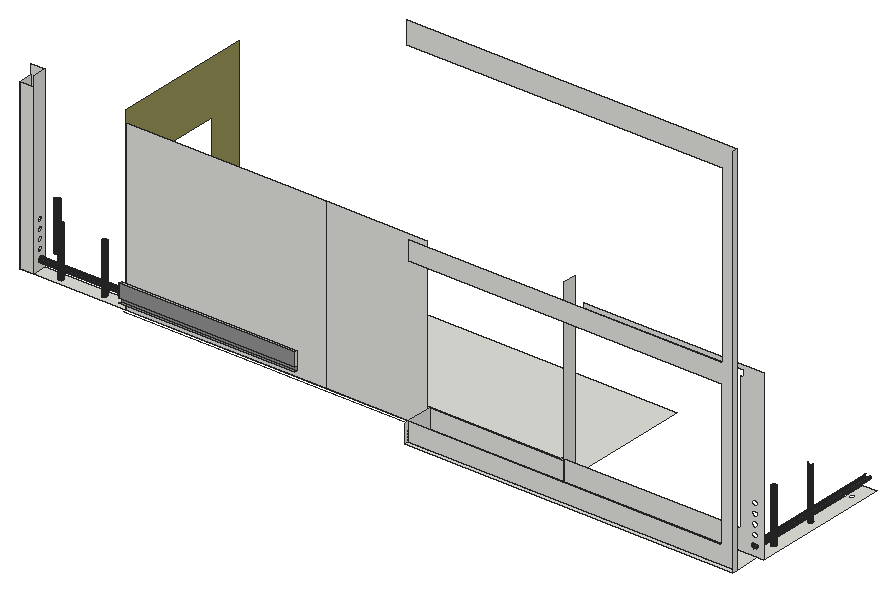
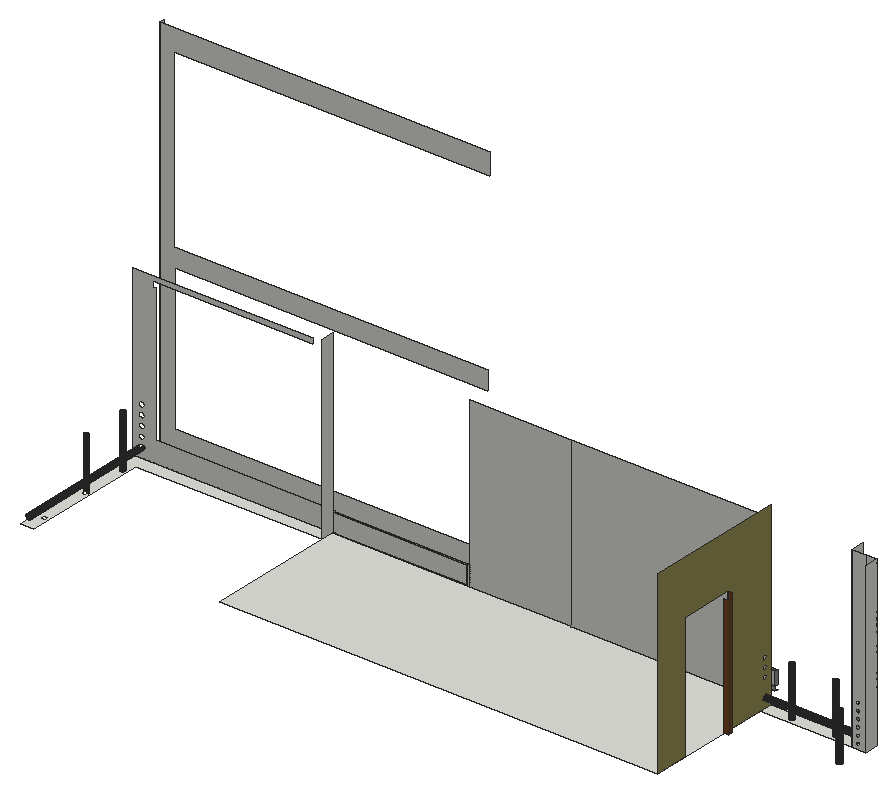
# SketchUp Ruby script. Lengths in inches.
U = 1.inch
M = Sketchup.active_model
def pt(a) = Geom::Point3d.new(a.map { |v| v * U })
def face(e, loops, mat)
  f = e.add_face(loops[0].map { |a| pt(a) })
  loops[1..].each { |l| e.add_face(l.map { |a| pt(a) }).erase! }
  f.material = f.back_material = mat if mat
  f
end
# faces: each face lists its corners as indices into pts; further lists are holes
def faces(e, pts, list, mat = nil) = list.each { |f| face(e, (f[0].is_a?(Array) ? f : [f]).map { |l| l.map { |i| pts[i] } }, mat) }
# xy, xz, yz: faces in a plane at the given z, y or x. An outline is a flat list of corners, or four numbers for a rectangle; further outlines are holes
def ring(l) = l.size == 4 ? [[l[0], l[1]], [l[2], l[1]], [l[2], l[3]], [l[0], l[3]]] : l.each_slice(2).to_a
def flat(e, list, mat, &to3) = list.each { |f| face(e, (f[0].is_a?(Array) ? f : [f]).map { |l| ring(l).map { |u, v| to3.(u, v) } }, mat) }
def xy(e, z, list, mat = nil) = flat(e, list, mat) { |x, y| [x, y, z] }
def xz(e, y, list, mat = nil) = flat(e, list, mat) { |x, z| [x, y, z] }
def yz(e, x, list, mat = nil) = flat(e, list, mat) { |y, z| [x, y, z] }
def lines(e, pts, list) = list.each { |a, b| e.add_line(pt(pts[a]), pt(pts[b])) }
# prism: a flat outline (further loops are holes) pulled along v
def prism(e, loops, v, mat = nil)
  f = face(e, loops, mat); d = Geom::Vector3d.new(v.map { |x| x * U })
  f.pushpull(f.normal.samedirection?(d) ? d.length : -d.length)
end
def box(e, o, s, mat = nil) = prism(e, [[o, [o[0] + s[0], o[1], o[2]], [o[0] + s[0], o[1] + s[1], o[2]], [o[0], o[1] + s[1], o[2]]]], [0, 0, s[2]], mat)
def at(x, y, z, deg = 0) = Geom::Transformation.translation(pt([x, y, z])) * Geom::Transformation.rotation(ORIGIN, Z_AXIS, deg.degrees)
def axes(o, x, y, z) = Geom::Transformation.new([*x, 0, *y, 0, *z, 0, *pt(o).to_a, 1])
def part(name) = M.definitions.add(name)
# library, detail: a bought-in or finely detailed component or shape, given as its bounding box
def library(name, o, s) = part(name).tap { |d| box(d.entities, o, s) }
def detail(e, o, s) = box(e.add_group.entities, o, s)
def put(e, d, t, mat = nil) = e.add_instance(d, t).tap { |i| i.material = mat if mat }
def group(e, t, mat = nil) = e.add_group.tap { |g| g.transformation = t; g.material = mat if mat }.entities
root = M.entities
M.materials.add("[0057_DarkKhaki]").color = [150, 145, 85]
M.materials.add("[0137_Black]").color = [71, 71, 71]
M.materials.add("[Color M05]").color = [145, 145, 145]
M.materials.add("[Wood Veneer 01]").color = [120, 70, 37]
xy(root,123,[[11.875,22.0625,20.875,31.0625],[[20.875,22.0625,82.85,31.0625],[35.53,25.16,35.13,25.24,34.76,25.43,34.46,25.7,34.23,26.04,34.1,26.42,34.08,26.83,34.16,27.23,34.34,27.59,34.61,27.9,34.95,28.125,35.34,28.25,35.75,28.28,36.15,28.2,36.51,28.02,36.82,27.75,37.04,27.41,37.17,27.02,37.2,26.61,37.11,26.21,36.93,25.85,36.66,25.54,36.32,25.32,35.9375,25.1875],[64.53,25.16,64.13,25.24,63.76,25.43,63.46,25.7,63.23,26.04,63.1,26.42,63.08,26.83,63.16,27.23,63.34,27.59,63.61,27.9,63.95,28.125,64.34,28.25,64.75,28.28,65.15,28.2,65.51,28.02,65.82,27.75,66.04,27.41,66.17,27.02,66.2,26.61,66.11,26.21,65.93,25.85,65.66,25.54,65.32,25.32,64.9375,25.1875]],[82.85,22.0625,376.99,116.75],[[376.99,22.0625,510.6875,22.0625,510.6875,116.75,501.6875,116.75,501.6875,31.0625,376.99,31.0625],[504.72,36.55,504.27,36.6,503.85,36.78,503.49,37.06,503.21,37.42,503.03,37.84,502.97,38.3,503.03,38.75,503.21,39.17,503.49,39.53,503.85,39.8125,504.27,39.99,504.72,40.05,505.18,39.99,505.6,39.8125,505.96,39.53,506.24,39.17,506.41,38.75,506.47,38.3,506.41,37.84,506.24,37.42,505.96,37.06,505.6,36.78,505.18,36.6],[504.72,67.92,504.27,67.98,503.85,68.15,503.49,68.43,503.21,68.8,503.03,69.22,502.97,69.67,503.03,70.125,503.21,70.55,503.49,70.91,503.85,71.1875,504.27,71.36,504.72,71.42,505.18,71.36,505.6,71.1875,505.96,70.91,506.24,70.55,506.41,70.125,506.47,69.67,506.41,69.22,506.24,68.8,505.96,68.43,505.6,68.15,505.18,67.98],[504.72,102.17,504.27,102.23,503.85,102.4,503.49,102.68,503.21,103.05,503.03,103.47,502.97,103.92,503.03,104.375,503.21,104.8,503.49,105.16,503.85,105.4375,504.27,105.61,504.72,105.67,505.18,105.61,505.6,105.4375,505.96,105.16,506.24,104.8,506.41,104.375,506.47,103.92,506.41,103.47,506.24,103.05,505.96,102.68,505.6,102.4,505.18,102.23]],[79.85,58.11,82.85,61.11]])
xy(root,123.19,[[286.64,1.0625,507.04,4.0625],[286.64,4.0625,507.04,22.0625]])
xy(root,129.65,[[82.85,16.375,200.79,18.1875]],"[Color M05]")
xy(root,132.55,[[82.85,16.375,200.79,18.1875]])
xz(root,4.0625,[[286.64,123.19,507.04,123.19,507.04,376.42,285.64,376.42,285.64,361.64,497.49,361.64,497.49,244.84,286.99,244.84,286.99,232.22,497.29,232.22,497.29,135.48,286.64,135.48]])
xz(root,16.375,[[82.85,132.55,200.79,141.65]],"[Color M05]")
xz(root,18.1875,[[82.85,132.55,200.79,141.65]])
xz(root,18.1875,[[82.85,129.65,200.79,132.55]],"[Color M05]")
xz(root,22.0625,[[11.875,123,20.875,235.42],[82.85,123,216.73,235.42],[216.73,123,216.79,235.42],[216.79,123,284.41,235.42],[284.41,123,376.99,123,376.99,123.19,286.64,123.19,286.64,135.48,376.99,135.48,376.99,137.03,375.29,137.03,375.29,135.98,284.41,135.98],
  [[376.99,123,376.99,137.03,495.71,137.03,495.71,228.47,497.29,228.47,497.29,232.22,390.0625,232.22,390.0625,235.42,510.6875,235.42,510.6875,123],[504.95,127.5625,505.43,127.625,505.88,127.8125,506.27,128.11,506.57,128.5,506.76,128.95,506.82,129.4375,506.76,129.92,506.57,130.375,506.27,130.76,505.88,131.0625,505.43,131.25,504.95,131.3125,504.46,131.25,504.01,131.0625,503.62,130.76,503.32,130.375,503.14,129.92,503.07,129.4375,503.14,128.95,503.32,128.5,503.62,128.11,504.01,127.8125,504.46,127.625],[504.95,134,505.43,134.0625,505.88,134.25,506.27,134.55,506.57,134.9375,506.76,135.39,506.82,135.875,506.76,136.36,506.57,136.8125,506.27,137.2,505.88,137.5,505.43,137.69,504.95,137.75,504.46,137.69,504.01,137.5,503.62,137.2,503.32,136.8125,503.14,136.36,503.07,135.875,503.14,135.39,503.32,134.9375,503.62,134.55,504.01,134.25,504.46,134.0625],[504.95,140.4375,505.43,140.5,505.88,140.6875,506.27,140.99,506.57,141.375,506.76,141.83,506.82,142.3125,506.76,142.8,506.57,143.25,506.27,143.64,505.88,143.9375,505.43,144.12,504.95,144.1875,504.46,144.12,504.01,143.9375,503.62,143.64,503.32,143.25,503.14,142.8,503.07,142.3125,503.14,141.83,503.32,141.375,503.62,140.99,504.01,140.6875,504.46,140.5],[504.95,146.875,505.43,146.9375,505.88,147.125,506.27,147.42,506.57,147.8125,506.76,148.26,506.82,148.75,506.76,149.23,506.57,149.6875,506.27,150.08,505.88,150.375,505.43,150.56,504.95,150.625,504.46,150.56,504.01,150.375,503.62,150.08,503.32,149.6875,503.14,149.23,503.07,148.75,503.14,148.26,503.32,147.8125,503.62,147.42,504.01,147.125,504.46,146.9375],[504.95,153.3125,505.43,153.375,505.88,153.5625,506.27,153.86,506.57,154.25,506.76,154.7,506.82,155.1875,506.76,155.67,506.57,156.125,506.27,156.51,505.88,156.8125,505.43,157,504.95,157.0625,504.46,157,504.01,156.8125,503.62,156.51,503.32,156.125,503.14,155.67,503.07,155.1875,503.14,154.7,503.32,154.25,503.62,153.86,504.01,153.5625,504.46,153.375]],[286.64,123.19,376.99,135.48]])
xz(root,31.0625,[[[11.875,123,20.875,242.04],[17.02,125.05,17.375,125.1,17.71,125.24,17.99,125.46,18.21,125.74,18.35,126.07,18.4,126.43,18.35,126.79,18.21,127.12,17.99,127.4,17.71,127.62,17.375,127.76,17.02,127.8,16.66,127.76,16.33,127.62,16.05,127.4,15.83,127.12,15.69,126.79,15.65,126.43,15.69,126.07,15.83,125.74,16.05,125.46,16.33,125.24,16.66,125.1],[17.02,129.99,17.375,130.04,17.71,130.18,17.99,130.39,18.21,130.68,18.35,131.01,18.4,131.37,18.35,131.72,18.21,132.05,17.99,132.34,17.71,132.56,17.375,132.69,17.02,132.74,16.66,132.69,16.33,132.56,16.05,132.34,15.83,132.05,15.69,131.72,15.65,131.37,15.69,131.01,15.83,130.68,16.05,130.39,16.33,130.18,16.66,130.04],[17.02,134.93,17.375,134.98,17.71,135.11,17.99,135.33,18.21,135.62,18.35,135.95,18.4,136.3,18.35,136.66,18.21,136.99,17.99,137.28,17.71,137.49,17.375,137.63,17.02,137.68,16.66,137.63,16.33,137.49,16.05,137.28,15.83,136.99,15.69,136.66,15.65,136.3,15.69,135.95,15.83,135.62,16.05,135.33,16.33,135.11,16.66,134.98],[17.02,139.87,17.375,139.91,17.71,140.05,17.99,140.27,18.21,140.55,18.35,140.89,18.4,141.24,18.35,141.6,18.21,141.93,17.99,142.21,17.71,142.43,17.375,142.57,17.02,142.62,16.66,142.57,16.33,142.43,16.05,142.21,15.83,141.93,15.69,141.6,15.65,141.24,15.69,140.89,15.83,140.55,16.05,140.27,16.33,140.05,16.66,139.91],[17.02,144.8,17.375,144.85,17.71,144.99,17.99,145.21,18.21,145.49,18.35,145.82,18.4,146.18,18.35,146.54,18.21,146.87,17.99,147.15,17.71,147.37,17.375,147.51,17.02,147.55,16.66,147.51,16.33,147.37,16.05,147.15,15.83,146.87,15.69,146.54,15.65,146.18,15.69,145.82,15.83,145.49,16.05,145.21,16.33,144.99,16.66,144.85],[17.02,149.74,17.375,149.79,17.71,149.93,17.99,150.14,18.21,150.43,18.35,150.76,18.4,151.12,18.35,151.47,18.21,151.8,17.99,152.09,17.71,152.31,17.375,152.44,17.02,152.49,16.66,152.44,16.33,152.31,16.05,152.09,15.83,151.8,15.69,151.47,15.65,151.12,15.69,150.76,15.83,150.43,16.05,150.14,16.33,149.93,16.66,149.79]]])
xz(root,58.11,[[79.85,123,82.85,207]],"[Wood Veneer 01]")
xz(root,61.11,[[79.85,123,82.85,204]],"[Wood Veneer 01]")
yz(root,11.875,[[22.0625,123,31.0625,235.42]])
yz(root,20.875,[[[22.0625,123,31.0625,242.04],[27.125,127.9375,26.6875,127.99,26.28,128.16,25.93,128.43,25.66,128.78,25.49,129.1875,25.4375,129.625,25.49,130.06,25.66,130.47,25.93,130.82,26.28,131.08,26.6875,131.25,27.125,131.3125,27.5625,131.25,27.97,131.08,28.32,130.82,28.59,130.47,28.75,130.06,28.8125,129.625,28.75,129.1875,28.59,128.78,28.32,128.43,27.97,128.16,27.5625,127.99],[27.125,133.9375,26.6875,133.99,26.28,134.16,25.93,134.43,25.66,134.78,25.49,135.1875,25.4375,135.625,25.49,136.06,25.66,136.47,25.93,136.82,26.28,137.08,26.6875,137.25,27.125,137.3125,27.5625,137.25,27.97,137.08,28.32,136.82,28.59,136.47,28.75,136.06,28.8125,135.625,28.75,135.1875,28.59,134.78,28.32,134.43,27.97,134.16,27.5625,133.99],[27.125,139.9375,26.6875,139.99,26.28,140.16,25.93,140.43,25.66,140.78,25.49,141.1875,25.4375,141.625,25.49,142.06,25.66,142.47,25.93,142.82,26.28,143.08,26.6875,143.25,27.125,143.3125,27.5625,143.25,27.97,143.08,28.32,142.82,28.59,142.47,28.75,142.06,28.8125,141.625,28.75,141.1875,28.59,140.78,28.32,140.43,27.97,140.16,27.5625,139.99],[27.125,145.9375,26.6875,145.99,26.28,146.16,25.93,146.43,25.66,146.78,25.49,147.1875,25.4375,147.625,25.49,148.06,25.66,148.47,25.93,148.82,26.28,149.08,26.6875,149.25,27.125,149.3125,27.5625,149.25,27.97,149.08,28.32,148.82,28.59,148.47,28.75,148.06,28.8125,147.625,28.75,147.1875,28.59,146.78,28.32,146.43,27.97,146.16,27.5625,145.99],[27.125,151.9375,26.6875,151.99,26.28,152.16,25.93,152.43,25.66,152.78,25.49,153.1875,25.4375,153.625,25.49,154.06,25.66,154.47,25.93,154.82,26.28,155.08,26.6875,155.25,27.125,155.3125,27.5625,155.25,27.97,155.08,28.32,154.82,28.59,154.47,28.75,154.06,28.8125,153.625,28.75,153.1875,28.59,152.78,28.32,152.43,27.97,152.16,27.5625,151.99]]])
yz(root,82.85,[[[22.0625,123,22.0625,243,116.75,243,116.75,123,94.11,123,94.11,207,58.11,207,58.11,123],[27.125,151.9375,27.5625,151.99,27.97,152.16,28.32,152.43,28.59,152.78,28.75,153.1875,28.8125,153.625,28.75,154.06,28.59,154.47,28.32,154.82,27.97,155.08,27.5625,155.25,27.125,155.3125,26.6875,155.25,26.28,155.08,25.93,154.82,25.66,154.47,25.49,154.06,25.4375,153.625,25.49,153.1875,25.66,152.78,25.93,152.43,26.28,152.16,26.6875,151.99],[27.125,145.9375,27.5625,145.99,27.97,146.16,28.32,146.43,28.59,146.78,28.75,147.1875,28.8125,147.625,28.75,148.06,28.59,148.47,28.32,148.82,27.97,149.08,27.5625,149.25,27.125,149.3125,26.6875,149.25,26.28,149.08,25.93,148.82,25.66,148.47,25.49,148.06,25.4375,147.625,25.49,147.1875,25.66,146.78,25.93,146.43,26.28,146.16,26.6875,145.99],[27.125,139.9375,27.5625,139.99,27.97,140.16,28.32,140.43,28.59,140.78,28.75,141.1875,28.8125,141.625,28.75,142.06,28.59,142.47,28.32,142.82,27.97,143.08,27.5625,143.25,27.125,143.3125,26.6875,143.25,26.28,143.08,25.93,142.82,25.66,142.47,25.49,142.06,25.4375,141.625,25.49,141.1875,25.66,140.78,25.93,140.43,26.28,140.16,26.6875,139.99],[27.125,127.9375,27.5625,127.99,27.97,128.16,28.32,128.43,28.59,128.78,28.75,129.1875,28.8125,129.625,28.75,130.06,28.59,130.47,28.32,130.82,27.97,131.08,27.5625,131.25,27.125,131.3125,26.6875,131.25,26.28,131.08,25.93,130.82,25.66,130.47,25.49,130.06,25.4375,129.625,25.49,129.1875,25.66,128.78,25.93,128.43,26.28,128.16,26.6875,127.99]]],"[0057_DarkKhaki]")
yz(root,82.85,[[16.375,132.55,18.1875,141.65]],"[Color M05]")
yz(root,200.79,[[16.375,132.55,18.1875,141.65]])
yz(root,286.64,[[1.0625,123.19,4.0625,135.48],[4.0625,123.19,22.0625,135.48]])
yz(root,376.99,[[22.0625,123,31.0625,243]])
yz(root,507.04,[[1.0625,123.19,4.0625,376.42]])
p = [[34.76,25.43,123],[35.13,25.24,123],[35.13,25.24,156.3125],[34.76,25.43,156.3125],[35.53,25.16,123],[35.53,25.16,156.3125],
  [35.9375,25.1875,123],[35.9375,25.1875,156.3125],[36.32,25.32,123],[36.32,25.32,156.3125],[63.76,25.43,123],[64.13,25.24,123],
  [64.13,25.24,156.3125],[63.76,25.43,156.3125],[64.53,25.16,123],[64.53,25.16,156.3125],[64.9375,25.1875,123],[64.9375,25.1875,156.3125],
  [65.32,25.32,123],[65.32,25.32,156.3125],[36.66,25.54,123],[36.66,25.54,156.3125],[65.66,25.54,123],[65.66,25.54,156.3125],
  [34.46,25.7,123],[34.46,25.7,156.3125],[63.46,25.7,123],[63.46,25.7,156.3125],[36.93,25.85,123],[36.93,25.85,156.3125],
  [65.93,25.85,123],[65.93,25.85,156.3125],[34.23,26.04,123],[34.23,26.04,156.3125],[63.23,26.04,123],[63.23,26.04,156.3125],
  [37.11,26.21,123],[37.11,26.21,156.3125],[66.11,26.21,123],[66.11,26.21,156.3125],[34.1,26.42,123],[34.1,26.42,156.3125],
  [63.1,26.42,123],[63.1,26.42,156.3125],[37.2,26.61,123],[37.2,26.61,156.3125],[66.2,26.61,123],[66.2,26.61,156.3125],
  [34.08,26.83,123],[34.08,26.83,156.3125],[63.08,26.83,123],[63.08,26.83,156.3125],[37.17,27.02,123],[37.17,27.02,156.3125],
  [66.17,27.02,123],[66.17,27.02,156.3125],[34.16,27.23,123],[34.16,27.23,156.3125],[63.16,27.23,123],[63.16,27.23,156.3125],
  [37.04,27.41,123],[37.04,27.41,156.3125],[66.04,27.41,123],[66.04,27.41,156.3125],[34.34,27.59,123],[34.34,27.59,156.3125],
  [63.34,27.59,123],[63.34,27.59,156.3125],[36.82,27.75,123],[36.82,27.75,156.3125],[65.82,27.75,123],[65.82,27.75,156.3125],
  [34.61,27.9,123],[34.61,27.9,156.3125],[63.61,27.9,123],[63.61,27.9,156.3125],[36.51,28.02,123],[36.51,28.02,156.3125],
  [65.51,28.02,123],[65.51,28.02,156.3125],[34.95,28.125,123],[34.95,28.125,156.3125],[63.95,28.125,123],[63.95,28.125,156.3125],
  [36.15,28.2,123],[36.15,28.2,156.3125],[65.15,28.2,123],[65.15,28.2,156.3125],[35.34,28.25,123],[35.34,28.25,156.3125],
  [64.34,28.25,123],[64.34,28.25,156.3125],[35.75,28.28,123],[35.75,28.28,156.3125],[64.75,28.28,123],[64.75,28.28,156.3125],
  [504.27,36.6,123],[504.72,36.55,123],[504.72,36.55,158.25],[504.27,36.6,158.25],[505.18,36.6,123],[505.18,36.6,158.25],
  [503.85,36.78,123],[503.85,36.78,158.25],[505.6,36.78,123],[505.6,36.78,158.25],[503.49,37.06,123],[503.49,37.06,158.25],
  [505.96,37.06,123],[505.96,37.06,158.25],[503.21,37.42,123],[503.21,37.42,158.25],[506.24,37.42,123],[506.24,37.42,158.25],
  [503.03,37.84,123],[503.03,37.84,158.25],[506.41,37.84,123],[506.41,37.84,158.25],[502.97,38.3,123],[502.97,38.3,158.25],
  [506.47,38.3,123],[506.47,38.3,158.25],[503.03,38.75,123],[503.03,38.75,158.25],[506.41,38.75,123],[506.41,38.75,158.25],
  [503.21,39.17,123],[503.21,39.17,158.25],[506.24,39.17,123],[506.24,39.17,158.25],[503.49,39.53,123],[503.49,39.53,158.25],
  [505.96,39.53,123],[505.96,39.53,158.25],[503.85,39.8125,123],[503.85,39.8125,158.25],[505.6,39.8125,123],[505.6,39.8125,158.25],
  [504.27,39.99,123],[504.27,39.99,158.25],[505.18,39.99,123],[505.18,39.99,158.25],[504.72,40.05,123],[504.72,40.05,158.25],
  [15.46,45.87,123],[15.96,45.8,123],[15.96,45.8,154.6875],[15.46,45.87,154.6875],[16.47,45.87,123],[16.47,45.87,154.6875],
  [15,46.06,123],[15,46.06,154.6875],[16.93,46.06,123],[16.93,46.06,154.6875],[14.59,46.37,123],[14.59,46.37,154.6875],
  [17.33,46.37,123],[17.33,46.37,154.6875],[14.29,46.77,123],[14.29,46.77,154.6875],[17.64,46.77,123],[17.64,46.77,154.6875],
  [14.09,47.24,123],[14.09,47.24,154.6875],[17.84,47.24,123],[17.84,47.24,154.6875],[14.03,47.74,123],[14.03,47.74,154.6875],
  [17.9,47.74,123],[17.9,47.74,154.6875],[14.09,48.24,123],[14.09,48.24,154.6875],[17.84,48.24,123],[17.84,48.24,154.6875],
  [14.29,48.71,123],[14.29,48.71,154.6875],[17.64,48.71,123],[17.64,48.71,154.6875],[14.59,49.11,123],[14.59,49.11,154.6875],
  [17.33,49.11,123],[17.33,49.11,154.6875],[15,49.41,123],[15,49.41,154.6875],[16.93,49.41,123],[16.93,49.41,154.6875],
  [15.46,49.61,123],[15.46,49.61,154.6875],[16.47,49.61,123],[16.47,49.61,154.6875],[15.96,49.67,123],[15.96,49.67,154.6875],
  [504.27,67.98,123],[504.72,67.92,123],[504.72,67.92,158.25],[504.27,67.98,158.25],[505.18,67.98,123],[505.18,67.98,158.25],
  [503.85,68.15,123],[503.85,68.15,158.25],[505.6,68.15,123],[505.6,68.15,158.25],[503.49,68.43,123],[503.49,68.43,158.25],
  [505.96,68.43,123],[505.96,68.43,158.25],[503.21,68.8,123],[503.21,68.8,158.25],[506.24,68.8,123],[506.24,68.8,158.25],
  [503.03,69.22,123],[503.03,69.22,158.25],[506.41,69.22,123],[506.41,69.22,158.25],[504.46,22.0625,127.625],[504.01,22.0625,127.8125],
  [504.01,116.75,127.8125],[504.46,116.75,127.625],[504.95,22.0625,127.5625],[504.95,116.75,127.5625],[505.43,22.0625,127.625],[505.43,116.75,127.625],
  [505.88,22.0625,127.8125],[505.88,116.75,127.8125],[503.62,22.0625,128.11],[503.62,116.75,128.11],[506.27,22.0625,128.11],[506.27,116.75,128.11],
  [20.875,26.6875,127.99],[20.875,27.125,127.9375],[82.85,27.125,127.9375],[82.85,26.6875,127.99],[20.875,27.5625,127.99],[82.85,27.5625,127.99],
  [20.875,26.28,128.16],[82.85,26.28,128.16],[20.875,27.97,128.16],[82.85,27.97,128.16],[503.32,22.0625,128.5],[503.32,116.75,128.5],
  [506.57,22.0625,128.5],[506.57,116.75,128.5],[20.875,25.93,128.43],[82.85,25.93,128.43],[20.875,28.32,128.43],[82.85,28.32,128.43],
  [20.875,25.66,128.78],[82.85,25.66,128.78],[20.875,28.59,128.78],[82.85,28.59,128.78],[503.14,22.0625,128.95],[503.14,116.75,128.95],
  [506.76,22.0625,128.95],[506.76,116.75,128.95],[20.875,25.49,129.1875],[82.85,25.49,129.1875],[20.875,28.75,129.1875],[82.85,28.75,129.1875],
  [503.07,22.0625,129.4375],[503.07,116.75,129.4375],[506.82,22.0625,129.4375],[506.82,116.75,129.4375],[20.875,25.4375,129.625],[82.85,25.4375,129.625],
  [20.875,28.8125,129.625],[82.85,28.8125,129.625],[503.14,22.0625,129.92],[503.14,116.75,129.92],[506.76,22.0625,129.92],[506.76,116.75,129.92],
  [20.875,25.49,130.06],[82.85,25.49,130.06],[20.875,28.75,130.06],[82.85,28.75,130.06],[503.32,22.0625,130.375],[503.32,116.75,130.375],
  [506.57,22.0625,130.375],[506.57,116.75,130.375],[20.875,25.66,130.47],[82.85,25.66,130.47],[20.875,28.59,130.47],[82.85,28.59,130.47],
  [503.62,22.0625,130.76],[503.62,116.75,130.76],[20.875,25.93,130.82],[82.85,25.93,130.82],[20.875,28.32,130.82],[82.85,28.32,130.82],
  [20.875,26.28,131.08],[82.85,26.28,131.08],[20.875,27.97,131.08],[82.85,27.97,131.08],[20.875,26.6875,131.25],[82.85,26.6875,131.25],
  [20.875,27.5625,131.25],[82.85,27.5625,131.25],[20.875,27.125,131.3125],[82.85,27.125,131.3125],[82.85,19.75,123],[376.99,19.75,123],
  [376.99,22.0625,123]]
faces(root,p,[[0,1,2,3],[1,4,5,2],[4,6,7,5],[6,8,9,7],[10,11,12,13],[11,14,15,12],[14,16,17,15],[16,18,19,17],
  [8,20,21,9],[18,22,23,19],[24,0,3,25],[26,10,13,27],[20,28,29,21],[22,30,31,23],[32,24,25,33],[34,26,27,35],
  [28,36,37,29],[30,38,39,31],[40,32,33,41],[42,34,35,43],[36,44,45,37],[38,46,47,39],[48,40,41,49],[50,42,43,51],
  [44,52,53,45],[46,54,55,47],[56,48,49,57],[58,50,51,59],[52,60,61,53],[54,62,63,55],[64,56,57,65],[66,58,59,67],
  [60,68,69,61],[62,70,71,63],[72,64,65,73],[74,66,67,75],[68,76,77,69],[70,78,79,71],[80,72,73,81],[82,74,75,83],
  [76,84,85,77],[78,86,87,79],[88,80,81,89],[90,82,83,91],[84,92,93,85],[86,94,95,87],[92,88,89,93],[94,90,91,95],
  [96,97,98,99],[97,100,101,98],[102,96,99,103],[100,104,105,101],[106,102,103,107],[104,108,109,105],[110,106,107,111],[108,112,113,109],
  [114,110,111,115],[112,116,117,113],[118,114,115,119],[116,120,121,117],[122,118,119,123],[120,124,125,121],[126,122,123,127],[124,128,129,125],
  [130,126,127,131],[128,132,133,129],[134,130,131,135],[132,136,137,133],[138,134,135,139],[136,140,141,137],[142,138,139,143],[140,142,143,141],
  [144,145,146,147],[145,148,149,146],[150,144,147,151],[148,152,153,149],[154,150,151,155],[152,156,157,153],[158,154,155,159],[156,160,161,157],
  [162,158,159,163],[160,164,165,161],[166,162,163,167],[164,168,169,165],[170,166,167,171],[168,172,173,169],[174,170,171,175],[172,176,177,173],
  [178,174,175,179],[176,180,181,177],[182,178,179,183],[180,184,185,181],[186,182,183,187],[184,188,189,185],[190,186,187,191],[188,190,191,189],
  [192,193,194,195],[193,196,197,194],[198,192,195,199],[196,200,201,197],[202,198,199,203],[200,204,205,201],[206,202,203,207],[204,208,209,205],
  [210,206,207,211],[208,212,213,209],[214,215,216,217],[218,214,217,219],[220,218,219,221],[222,220,221,223],[215,224,225,216],[226,222,223,227],
  [228,229,230,231],[229,232,233,230],[234,228,231,235],[232,236,237,233],[224,238,239,225],[240,226,227,241],[242,234,235,243],[236,244,245,237],
  [246,242,243,247],[244,248,249,245],[238,250,251,239],[252,240,241,253],[254,246,247,255],[248,256,257,249],[250,258,259,251],[260,252,253,261],
  [262,254,255,263],[256,264,265,257],[258,266,267,259],[268,260,261,269],[270,262,263,271],[264,272,273,265],[266,274,275,267],[276,268,269,277],
  [278,270,271,279],[272,280,281,273],[274,282,283,275],[284,278,279,285],[280,286,287,281],[288,284,285,289],[286,290,291,287],[292,288,289,293],
  [290,294,295,291],[296,292,293,297],[294,296,297,295]],"[0137_Black]")
lines(root,p,[[298,299],[300,299]])
